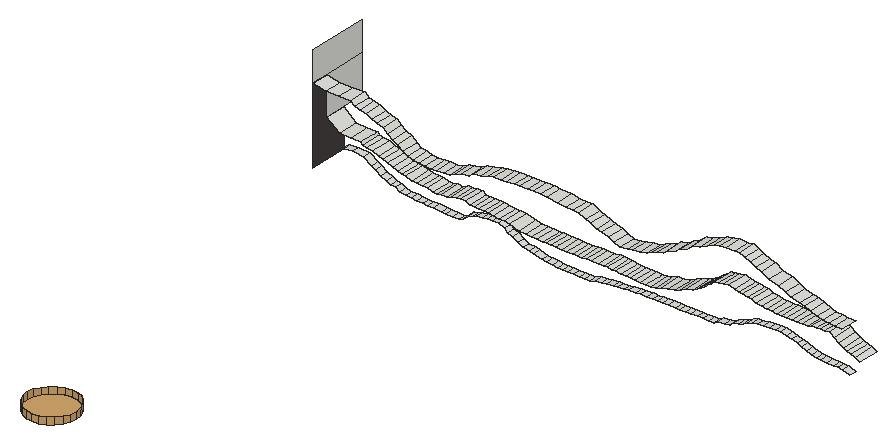
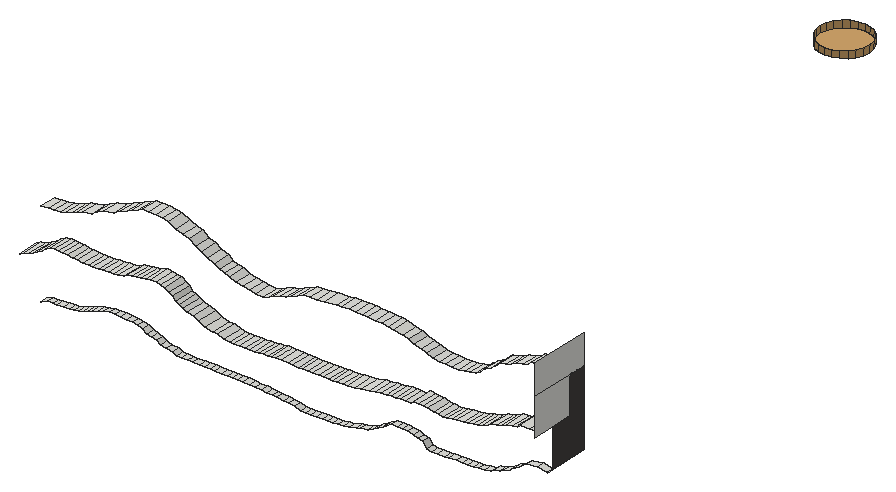
# SketchUp Ruby script. Lengths in inches.
U = 1.inch
M = Sketchup.active_model
def pt(a) = Geom::Point3d.new(a.map { |v| v * U })
def face(e, loops, mat)
  f = e.add_face(loops[0].map { |a| pt(a) })
  loops[1..].each { |l| e.add_face(l.map { |a| pt(a) }).erase! }
  f.material = f.back_material = mat if mat
  f
end
# faces: each face lists its corners as indices into pts; further lists are holes
def faces(e, pts, list, mat = nil) = list.each { |f| face(e, (f[0].is_a?(Array) ? f : [f]).map { |l| l.map { |i| pts[i] } }, mat) }
# xy, xz, yz: faces in a plane at the given z, y or x. An outline is a flat list of corners, or four numbers for a rectangle; further outlines are holes
def ring(l) = l.size == 4 ? [[l[0], l[1]], [l[2], l[1]], [l[2], l[3]], [l[0], l[3]]] : l.each_slice(2).to_a
def flat(e, list, mat, &to3) = list.each { |f| face(e, (f[0].is_a?(Array) ? f : [f]).map { |l| ring(l).map { |u, v| to3.(u, v) } }, mat) }
def xy(e, z, list, mat = nil) = flat(e, list, mat) { |x, y| [x, y, z] }
def xz(e, y, list, mat = nil) = flat(e, list, mat) { |x, z| [x, y, z] }
def yz(e, x, list, mat = nil) = flat(e, list, mat) { |y, z| [x, y, z] }
def lines(e, pts, list) = list.each { |a, b| e.add_line(pt(pts[a]), pt(pts[b])) }
# prism: a flat outline (further loops are holes) pulled along v
def prism(e, loops, v, mat = nil)
  f = face(e, loops, mat); d = Geom::Vector3d.new(v.map { |x| x * U })
  f.pushpull(f.normal.samedirection?(d) ? d.length : -d.length)
end
def box(e, o, s, mat = nil) = prism(e, [[o, [o[0] + s[0], o[1], o[2]], [o[0] + s[0], o[1] + s[1], o[2]], [o[0], o[1] + s[1], o[2]]]], [0, 0, s[2]], mat)
def at(x, y, z, deg = 0) = Geom::Transformation.translation(pt([x, y, z])) * Geom::Transformation.rotation(ORIGIN, Z_AXIS, deg.degrees)
def axes(o, x, y, z) = Geom::Transformation.new([*x, 0, *y, 0, *z, 0, *pt(o).to_a, 1])
def part(name) = M.definitions.add(name)
# library, detail: a bought-in or finely detailed component or shape, given as its bounding box
def library(name, o, s) = part(name).tap { |d| box(d.entities, o, s) }
def detail(e, o, s) = box(e.add_group.entities, o, s)
def put(e, d, t, mat = nil) = e.add_instance(d, t).tap { |i| i.material = mat if mat }
def group(e, t, mat = nil) = e.add_group.tap { |g| g.transformation = t; g.material = mat if mat }.entities
root = M.entities
M.materials.add("[Field Square Tile]").color = [211, 167, 108]
M.materials.add("[Granite Tile]1").color = [68, 65, 63]
xy(root,237.65,[[2039.58,2401.37,2040.27,2402.3],[2040.27,2401.37,2040.89,2402.3]])
xy(root,238.33,[[2048.68,2401.37,2049.23,2402.3],[2049.23,2401.37,2049.91,2402.3]])
xy(root,238.34,[[2050.59,2401.37,2051.52,2402.3],[2051.52,2401.37,2052.01,2402.3],[2052.01,2401.37,2052.77,2402.3],[2052.77,2401.37,2053.4,2402.3],[2053.4,2401.37,2054.15,2402.3],
  [2054.15,2401.37,2054.77,2402.3],[2054.77,2401.37,2055.54,2402.3],[2055.54,2401.37,2056.16,2402.3]])
xy(root,241.52,[[2010.28,2396.68,2010.34,2402.3]])
xy(root,241.68,[[2040.78,2398.8,2041.37,2401.37]])
xy(root,241.75,[[2043.13,2398.8,2044,2401.37],[2044,2398.8,2044.62,2401.37],[2044.62,2398.8,2045.13,2401.37]])
xy(root,250.6875,[[2030.6,2327.89,2029.81,2328,2029.07,2328.3,2028.43,2328.79,2027.95,2329.43,2027.64,2330.16,2027.54,2330.96,2027.64,2331.75,2027.95,2332.49,2028.43,2333.12,2029.07,2333.61,2029.81,2333.91,2030.6,2334.02,2031.39,2333.91,2032.13,2333.61,2032.76,2333.12,2033.25,2332.49,2033.56,2331.75,2033.66,2330.96,2033.56,2330.16,2033.25,2329.43,2032.76,2328.79,2032.13,2328.3,2031.39,2328]],"[Field Square Tile]")
xz(root,2396.68,[[2010.28,241.52,2010.34,251.5]])
yz(root,2010.34,[[2398.8,246.2,2404.3,250.88],[2396.68,250.88,2404.3,254.5]])
yz(root,2010.34,[[2396.68,241.52,2401.37,241.52,2401.37,246.2,2398.8,246.2,2398.8,250.88,2396.68,250.88]],"[Granite Tile]1")
p = [[2040.89,2401.37,237.65],[2040.89,2402.3,237.65],[2041.56,2402.3,237.89],[2041.56,2401.37,237.89],[2036.22,2401.37,237.76],[2036.22,2402.3,237.76],
  [2036.93,2402.3,237.71],[2036.93,2401.37,237.71],[2037.54,2402.3,237.68],[2037.54,2401.37,237.68],[2038.14,2402.3,237.67],[2038.14,2401.37,237.67],
  [2038.89,2402.3,237.66],[2038.89,2401.37,237.66],[2039.58,2402.3,237.65],[2039.58,2401.37,237.65],[2034.87,2401.37,237.9],[2034.87,2402.3,237.9],
  [2035.53,2402.3,237.82],[2035.53,2401.37,237.82],[2033.93,2401.37,238.21],[2033.93,2402.3,238.21],[2042.32,2402.3,237.94],[2042.32,2401.37,237.94],
  [2042.9375,2402.3,237.98],[2042.9375,2401.37,237.98],[2043.79,2402.3,238.1],[2043.79,2401.37,238.1],[2044.34,2402.3,238.13],[2044.34,2401.37,238.13],
  [2045.1,2402.3,238.15],[2045.1,2401.37,238.15],[2033.46,2401.37,238.31],[2033.46,2402.3,238.31],[2045.73,2402.3,238.26],[2045.73,2401.37,238.26],
  [2032.55,2401.37,238.43],[2032.55,2402.3,238.43],[2046.48,2402.3,238.28],[2046.48,2401.37,238.28],[2047.11,2402.3,238.3],[2047.11,2401.37,238.3],
  [2047.96,2402.3,238.32],[2047.96,2401.37,238.32],[2048.68,2402.3,238.33],[2048.68,2401.37,238.33],[2049.91,2401.37,238.33],[2049.91,2402.3,238.33],
  [2050.59,2402.3,238.34],[2050.59,2401.37,238.34],[2056.16,2401.37,238.34],[2056.16,2402.3,238.34],[2056.67,2402.3,238.59],[2056.67,2401.37,238.59],
  [2031.9,2401.37,238.74],[2031.9,2402.3,238.74],[2072.19,2401.37,238.78],[2072.19,2402.3,238.78],[2072.97,2402.3,238.43],[2072.97,2401.37,238.43],
  [2057.49,2402.3,238.72],[2057.49,2401.37,238.72],[2031.32,2401.37,239.11],[2031.32,2402.3,239.11],[2058.18,2402.3,238.86],[2058.18,2401.37,238.86],
  [2021.53,2401.37,238.92],[2021.53,2402.3,238.92],[2022.57,2402.3,238.82],[2022.57,2401.37,238.82],[2023.08,2402.3,238.8],[2023.08,2401.37,238.8],
  [2023.95,2402.3,238.79],[2023.95,2401.37,238.79],[2024.69,2402.3,238.77],[2024.69,2401.37,238.77],[2025.22,2402.3,238.9375],[2025.22,2401.37,238.9375],
  [2069.47,2401.37,238.875],[2069.47,2402.3,238.875],[2070.22,2402.3,238.83],[2070.22,2401.37,238.83],[2070.98,2402.3,238.8],[2070.98,2401.37,238.8],
  [2071.52,2402.3,238.79],[2071.52,2401.37,238.79],[2019.44,2401.37,238.97],[2019.44,2402.3,238.97],[2020.14,2402.3,238.94],[2020.14,2401.37,238.94],
  [2020.84,2402.3,238.93],[2020.84,2401.37,238.93],[2025.78,2402.3,239.55],[2025.78,2401.37,239.55],[2058.69,2402.3,239.18],[2058.69,2401.37,239.18],
  [2068.32,2401.37,239.04],[2068.32,2402.3,239.04],[2068.9,2402.3,238.94],[2068.9,2401.37,238.94],[2018.07,2401.37,239.09],[2018.07,2402.3,239.09],
  [2018.76,2402.3,239.03],[2018.76,2401.37,239.03],[2067.66,2401.37,239.29],[2067.66,2402.3,239.29],[2017.29,2401.37,239.19],[2017.29,2402.3,239.19],
  [2030.74,2401.37,239.38],[2030.74,2402.3,239.38],[2016.78,2401.37,239.52],[2016.78,2402.3,239.52],[2059.28,2402.3,239.35],[2059.28,2401.37,239.35],
  [2067.08,2401.37,239.53],[2067.08,2402.3,239.53],[2030.28,2401.37,239.71],[2030.28,2402.3,239.71],[2059.84,2402.3,239.52],[2059.84,2401.37,239.52],
  [2016.22,2401.37,239.64],[2016.22,2402.3,239.64],[2060.39,2402.3,239.85],[2060.39,2401.37,239.85],[2066.55,2401.37,239.7],[2066.55,2402.3,239.7],
  [2015.77,2401.37,239.86],[2015.77,2402.3,239.86],[2026.36,2402.3,239.69],[2026.36,2401.37,239.69],[2026.91,2402.3,239.88],[2026.91,2401.37,239.88],
  [2029.58,2401.37,240.11],[2029.58,2402.3,240.11],[2065.86,2401.37,239.92],[2065.86,2402.3,239.92],[2061.03,2402.3,240.03],[2061.03,2401.37,240.03],
  [2014.98,2401.37,240.2],[2014.98,2402.3,240.2],[2027.64,2402.3,239.99],[2027.64,2401.37,239.99],[2065.23,2401.37,240.11],[2065.23,2402.3,240.11],
  [2028.23,2402.3,240.05],[2028.23,2401.37,240.05],[2028.89,2402.3,240.09],[2028.89,2401.37,240.09],[2061.6875,2402.3,240.12],[2061.6875,2401.37,240.12],
  [2062.36,2402.3,240.19],[2062.36,2401.37,240.19],[2064.45,2401.37,240.27],[2064.45,2402.3,240.27],[2014.38,2401.37,240.59],[2014.38,2402.3,240.59],
  [2063.125,2402.3,240.23],[2063.125,2401.37,240.23],[2063.83,2402.3,240.25],[2063.83,2401.37,240.25],[2013.84,2401.37,240.85],[2013.84,2402.3,240.85],
  [2012.82,2401.37,241.55],[2012.82,2402.3,241.55],[2046.76,2398.8,241.57],[2046.76,2401.37,241.57],[2047.3,2401.37,241.53],[2047.3,2398.8,241.53],
  [2047.92,2401.37,241.51],[2047.92,2398.8,241.51],[2048.47,2401.37,241.49],[2048.47,2398.8,241.49],[2049.17,2401.37,241.48],[2049.17,2398.8,241.48],
  [2049.83,2401.37,241.47],[2049.83,2398.8,241.47],[2050.4,2401.37,241.46],[2050.4,2398.8,241.46],[2051.11,2401.37,241.6],[2051.11,2398.8,241.6],
  [2010.34,2401.37,241.52],[2010.34,2402.3,241.52],[2011.55,2402.3,241.69],[2011.55,2401.37,241.69],[2046.15,2398.8,241.66],[2046.15,2401.37,241.66],
  [2051.84,2401.37,241.85],[2051.84,2398.8,241.85],[2037.12,2398.8,241.75],[2037.12,2401.37,241.75],[2037.57,2401.37,241.74],[2037.57,2398.8,241.74],
  [2038.12,2401.37,241.72],[2038.12,2398.8,241.72],[2038.75,2401.37,241.71],[2038.75,2398.8,241.71],[2039.38,2401.37,241.7],[2039.38,2398.8,241.7],
  [2040.11,2401.37,241.69],[2040.11,2398.8,241.69],[2040.78,2401.37,241.68],[2040.78,2398.8,241.68],[2041.37,2398.8,241.68],[2041.37,2401.37,241.68],
  [2041.86,2401.37,241.67],[2041.86,2398.8,241.67],[2042.5625,2401.37,241.74],[2042.5625,2398.8,241.74],[2043.13,2401.37,241.75],[2043.13,2398.8,241.75],
  [2045.13,2398.8,241.75],[2045.13,2401.37,241.75],[2045.62,2401.37,241.67],[2045.62,2398.8,241.67],[2034.93,2398.8,241.89],[2034.93,2401.37,241.89],
  [2035.75,2401.37,241.83],[2035.75,2398.8,241.83],[2036.35,2401.37,241.78],[2036.35,2398.8,241.78],[2052.51,2401.37,241.91],[2052.51,2398.8,241.91],
  [2034.16,2398.8,241.96],[2034.16,2401.37,241.96],[2053.41,2401.37,242.1],[2053.41,2398.8,242.1],[2032.99,2398.8,242.24],[2032.99,2401.37,242.24],
  [2054.18,2401.37,242.46],[2054.18,2398.8,242.46],[2032.32,2398.8,242.34],[2032.32,2401.37,242.34],[2075.79,2398.8,242.51],[2075.79,2401.37,242.51],
  [2076.3,2401.37,242.21],[2076.3,2398.8,242.21],[2031.66,2398.8,242.38],[2031.66,2401.37,242.38],[2031,2398.8,242.48],[2031,2401.37,242.48],
  [2022.82,2398.8,242.68],[2022.82,2401.37,242.68],[2023.49,2401.37,242.51],[2023.49,2398.8,242.51],[2024.01,2401.37,242.46],[2024.01,2398.8,242.46],
  [2024.55,2401.37,242.58],[2024.55,2398.8,242.58],[2030.36,2398.8,242.57],[2030.36,2401.37,242.57],[2054.88,2401.37,242.78],[2054.88,2398.8,242.78],
  [2075.2,2398.8,242.68],[2075.2,2401.37,242.68],[2025.18,2401.37,242.57],[2025.18,2398.8,242.57],[2025.81,2401.37,242.81],[2025.81,2398.8,242.81],
  [2027.58,2398.8,242.92],[2027.58,2401.37,242.92],[2028.01,2401.37,242.625],[2028.01,2398.8,242.625],[2028.62,2401.37,242.65],[2028.62,2398.8,242.65],
  [2029.17,2401.37,242.62],[2029.17,2398.8,242.62],[2029.8,2401.37,242.58],[2029.8,2398.8,242.58],[2021.47,2398.8,242.78],[2021.47,2401.37,242.78],
  [2022.28,2401.37,242.73],[2022.28,2398.8,242.73],[2074.7,2398.8,242.875],[2074.7,2401.37,242.875],[2020.17,2398.8,243.06],[2020.17,2401.37,243.06],
  [2020.89,2401.37,242.85],[2020.89,2398.8,242.85],[2026.38,2401.37,242.86],[2026.38,2398.8,242.86],[2055.65,2401.37,242.97],[2055.65,2398.8,242.97],
  [2026.94,2401.37,242.89],[2026.94,2398.8,242.89],[2074.31,2398.8,243.09],[2074.31,2401.37,243.09],[2056.18,2401.37,243.23],[2056.18,2398.8,243.23],
  [2019.1,2398.8,243.3],[2019.1,2401.37,243.3],[2019.6875,2401.37,243.14],[2019.6875,2398.8,243.14],[2073.7,2398.8,243.43],[2073.7,2401.37,243.43],
  [2056.58,2401.37,243.48],[2056.58,2398.8,243.48],[2018.46,2398.8,243.48],[2018.46,2401.37,243.48],[2073.16,2398.8,243.8],[2073.16,2401.37,243.8],
  [2017.94,2398.8,243.79],[2017.94,2401.37,243.79],[2057.1,2401.37,243.72],[2057.1,2398.8,243.72],[2057.4375,2401.37,244.12],[2057.4375,2398.8,244.12],
  [2017.28,2398.8,243.95],[2017.28,2401.37,243.95],[2072.56,2398.8,244.18],[2072.56,2401.37,244.18],[2016.76,2398.8,244.11],[2016.76,2401.37,244.11],
  [2065.38,2398.8,243.99],[2065.38,2401.37,243.99],[2066.1,2401.37,243.95],[2066.1,2398.8,243.95],[2066.6,2401.37,243.93],[2066.6,2398.8,243.93],
  [2067.29,2401.37,243.91],[2067.29,2398.8,243.91],[2067.86,2401.37,243.89],[2067.86,2398.8,243.89],[2068.56,2401.37,243.88],[2068.56,2398.8,243.88],
  [2069.21,2401.37,243.94],[2069.21,2398.8,243.94],[2069.85,2401.37,243.95],[2069.85,2398.8,243.95],[2070.41,2401.37,244.1],[2070.41,2398.8,244.1],
  [2064.2,2398.8,244.11],[2064.2,2401.37,244.11],[2064.76,2401.37,244.04],[2064.76,2398.8,244.04],[2016.09,2398.8,244.41],[2016.09,2401.37,244.41],
  [2057.91,2401.37,244.39],[2057.91,2398.8,244.39],[2063.45,2398.8,244.25],[2063.45,2401.37,244.25],[2071.04,2401.37,244.13],[2071.04,2398.8,244.13],
  [2071.52,2401.37,244.15],[2071.52,2398.8,244.15],[2072.04,2401.37,244.17],[2072.04,2398.8,244.17],[2062.99,2398.8,244.51],[2062.99,2401.37,244.51],
  [2015.33,2398.8,244.54],[2015.33,2401.37,244.54],[2058.39,2401.37,244.73],[2058.39,2398.8,244.73],[2014.77,2398.8,244.61],[2014.77,2401.37,244.61],
  [2061.84,2398.8,244.67],[2061.84,2401.37,244.67],[2062.45,2401.37,244.55],[2062.45,2398.8,244.55],[2014.55,2398.8,244.92],[2014.55,2401.37,244.92],
  [2058.875,2401.37,244.87],[2058.875,2398.8,244.87],[2060.79,2398.8,244.81],[2060.79,2401.37,244.81],[2061.36,2401.37,244.7],[2061.36,2398.8,244.7],
  [2060.14,2398.8,245.01],[2060.14,2401.37,245.01],[2011.91,2398.8,244.96],[2011.91,2401.37,244.96],[2013.3,2401.37,244.9375],[2013.3,2398.8,244.9375],
  [2059.46,2401.37,244.95],[2059.46,2398.8,244.95],[2010.34,2398.8,246.2],[2010.34,2401.37,246.2],[2047.59,2396.68,246.35],[2047.59,2398.8,246.35],
  [2048.36,2398.8,246.05],[2048.36,2396.68,246.05],[2049.26,2398.8,246.13],[2049.26,2396.68,246.13],[2049.97,2398.8,246.29],[2049.97,2396.68,246.29],
  [2050.77,2398.8,246.41],[2050.77,2396.68,246.41],[2046.98,2396.68,246.66],[2046.98,2398.8,246.66],[2051.68,2398.8,246.55],[2051.68,2396.68,246.55],
  [2023.4,2396.68,246.62],[2023.4,2398.8,246.62],[2024.14,2398.8,246.54],[2024.14,2396.68,246.54],[2024.92,2398.8,246.51],[2024.92,2396.68,246.51],
  [2025.7,2398.8,246.58],[2025.7,2396.68,246.58],[2074.89,2396.68,246.59],[2074.89,2398.8,246.59],[2075.78,2398.8,246.55],[2075.78,2396.68,246.55],
  [2022.74,2396.68,246.73],[2022.74,2398.8,246.73],[2026.5,2398.8,246.59],[2026.5,2396.68,246.59],[2027.3,2398.8,246.69],[2027.3,2396.68,246.69],
  [2052.41,2398.8,246.92],[2052.41,2396.68,246.92],[2074.18,2396.68,246.66],[2074.18,2398.8,246.66],[2022.02,2396.68,246.88],[2022.02,2398.8,246.88],
  [2028.01,2398.8,247.03],[2028.01,2396.68,247.03],[2046.125,2396.68,246.94],[2046.125,2398.8,246.94],[2073.39,2396.68,246.75],[2073.39,2398.8,246.75],
  [2072.7,2396.68,246.95],[2072.7,2398.8,246.95],[2021.47,2396.68,247.25],[2021.47,2398.8,247.25],[2045.44,2396.68,247.08],[2045.44,2398.8,247.08],
  [2053.02,2398.8,247.12],[2053.02,2396.68,247.12],[2028.7,2398.8,247.2],[2028.7,2396.68,247.2],[2071.89,2396.68,247.25],[2071.89,2398.8,247.25],
  [2044.76,2396.68,247.46],[2044.76,2398.8,247.46],[2053.7,2398.8,247.31],[2053.7,2396.68,247.31],[2029.67,2398.8,247.39],[2029.67,2396.68,247.39],
  [2071.21,2396.68,247.53],[2071.21,2398.8,247.53],[2020.83,2396.68,247.72],[2020.83,2398.8,247.72],[2054.27,2398.8,247.71],[2054.27,2396.68,247.71],
  [2030.3,2398.8,247.78],[2030.3,2396.68,247.78],[2044.13,2396.68,247.66],[2044.13,2398.8,247.66],[2070.63,2396.68,247.66],[2070.63,2398.8,247.66],
  [2020.18,2396.68,248.07],[2020.18,2398.8,248.07],[2043.29,2396.68,248.08],[2043.29,2398.8,248.08],[2055.2,2398.8,248.03],[2055.2,2396.68,248.03],
  [2069.5,2396.68,247.9],[2069.5,2398.8,247.9],[2031.08,2398.8,247.89],[2031.08,2396.68,247.89],[2032.08,2398.8,248.18],[2032.08,2396.68,248.18],
  [2068.9,2396.68,248.26],[2068.9,2398.8,248.26],[2055.91,2398.8,248.46],[2055.91,2396.68,248.46],[2019.55,2396.68,248.51],[2019.55,2398.8,248.51],
  [2041.67,2396.68,248.15],[2041.67,2398.8,248.15],[2042.49,2398.8,248.11],[2042.49,2396.68,248.11],[2032.72,2398.8,248.29],[2032.72,2396.68,248.29],
  [2040.64,2396.68,248.28],[2040.64,2398.8,248.28],[2033.61,2398.8,248.35],[2033.61,2396.68,248.35],[2039.24,2396.68,248.39],[2039.24,2398.8,248.39],
  [2067.99,2396.68,248.69],[2067.99,2398.8,248.69],[2034.34,2398.8,248.4],[2034.34,2396.68,248.4],[2035.33,2398.8,248.4375],[2035.33,2396.68,248.4375],
  [2035.99,2398.8,248.46],[2035.99,2396.68,248.46],[2038.51,2396.68,248.49],[2038.51,2398.8,248.49],[2019.06,2396.68,249.01],[2019.06,2398.8,249.01],
  [2036.88,2398.8,248.47],[2036.88,2396.68,248.47],[2037.62,2398.8,248.48],[2037.62,2396.68,248.48],[2056.69,2398.8,248.82],[2056.69,2396.68,248.82],
  [2066.77,2396.68,248.95],[2066.77,2398.8,248.95],[2057.41,2398.8,249.37],[2057.41,2396.68,249.37],[2065.88,2396.68,249.46],[2065.88,2398.8,249.46],
  [2018.29,2396.68,249.2],[2018.29,2398.8,249.2],[2017.62,2396.68,249.41],[2017.62,2398.8,249.41],[2016.95,2396.68,249.8],[2016.95,2398.8,249.8],
  [2058.2,2398.8,249.5625],[2058.2,2396.68,249.5625],[2065.12,2396.68,249.68],[2065.12,2398.8,249.68],[2059.1,2398.8,249.9],[2059.1,2396.68,249.9],
  [2064.46,2396.68,250.0625],[2064.46,2398.8,250.0625],[2016.15,2396.68,249.97],[2016.15,2398.8,249.97],[2060.02,2398.8,250.35],[2060.02,2396.68,250.35],
  [2015.54,2396.68,250.15],[2015.54,2398.8,250.15],[2015.01,2396.68,250.55],[2015.01,2398.8,250.55],[2063.77,2396.68,250.32],[2063.77,2398.8,250.32],
  [2060.68,2398.8,250.49],[2060.68,2396.68,250.49],[2063.15,2396.68,250.61],[2063.15,2398.8,250.61],[2010.34,2396.68,250.88],[2010.34,2398.8,250.88],
  [2011.93,2398.8,250.53],[2011.93,2396.68,250.53],[2013.55,2398.8,250.54],[2013.55,2396.68,250.54],[2061.49,2398.8,250.6],[2061.49,2396.68,250.6],
  [2062.51,2398.8,250.58],[2062.51,2396.68,250.58],[2030.6,2327.89,251.5],[2029.81,2328,251.5],[2029.81,2328,250.6875],[2030.6,2327.89,250.6875],
  [2031.39,2328,251.5],[2031.39,2328,250.6875],[2029.07,2328.3,251.5],[2029.07,2328.3,250.6875],[2032.13,2328.3,251.5],[2032.13,2328.3,250.6875],
  [2028.43,2328.79,251.5],[2028.43,2328.79,250.6875],[2032.76,2328.79,251.5],[2032.76,2328.79,250.6875],[2027.95,2329.43,251.5],[2027.95,2329.43,250.6875],
  [2033.25,2329.43,251.5],[2033.25,2329.43,250.6875],[2027.64,2330.16,251.5],[2027.64,2330.16,250.6875],[2033.56,2330.16,251.5],[2033.56,2330.16,250.6875],
  [2027.54,2330.96,251.5],[2027.54,2330.96,250.6875],[2033.66,2330.96,251.5],[2033.66,2330.96,250.6875],[2027.64,2331.75,251.5],[2027.64,2331.75,250.6875],
  [2033.56,2331.75,251.5],[2033.56,2331.75,250.6875],[2027.95,2332.49,251.5],[2027.95,2332.49,250.6875],[2033.25,2332.49,251.5],[2033.25,2332.49,250.6875],
  [2028.43,2333.12,251.5],[2028.43,2333.12,250.6875],[2032.76,2333.12,251.5],[2032.76,2333.12,250.6875],[2029.07,2333.61,251.5],[2029.07,2333.61,250.6875],
  [2032.13,2333.61,251.5],[2032.13,2333.61,250.6875],[2029.81,2333.91,251.5],[2029.81,2333.91,250.6875],[2031.39,2333.91,251.5],[2031.39,2333.91,250.6875],
  [2030.6,2334.02,251.5],[2030.6,2334.02,250.6875]]
faces(root,p,[[0,1,2,3],[4,5,6,7],[7,6,8,9],[9,8,10,11],[11,10,12,13],[13,12,14,15],[16,17,18,19],[19,18,5,4],
  [20,21,17,16],[3,2,22,23],[23,22,24,25],[25,24,26,27],[27,26,28,29],[29,28,30,31],[32,33,21,20],[31,30,34,35],
  [36,37,33,32],[35,34,38,39],[39,38,40,41],[41,40,42,43],[43,42,44,45],[46,47,48,49],[50,51,52,53],[54,55,37,36],
  [56,57,58,59],[53,52,60,61],[62,63,55,54],[61,60,64,65],[66,67,68,69],[69,68,70,71],[71,70,72,73],[73,72,74,75],
  [75,74,76,77],[78,79,80,81],[81,80,82,83],[83,82,84,85],[85,84,57,56],[86,87,88,89],[89,88,90,91],[91,90,67,66],
  [77,76,92,93],[65,64,94,95],[96,97,98,99],[99,98,79,78],[100,101,102,103],[103,102,87,86],[104,105,97,96],[106,107,101,100],
  [108,109,63,62],[110,111,107,106],[95,94,112,113],[114,115,105,104],[116,117,109,108],[113,112,118,119],[120,121,111,110],[119,118,122,123],
  [124,125,115,114],[126,127,121,120],[93,92,128,129],[129,128,130,131],[132,133,117,116],[134,135,125,124],[123,122,136,137],[138,139,127,126],
  [131,130,140,141],[142,143,135,134],[141,140,144,145],[145,144,146,147],[137,136,148,149],[147,146,133,132],[149,148,150,151],[152,153,143,142],
  [154,155,139,138],[151,150,156,157],[157,156,158,159],[159,158,153,152],[160,161,155,154],[162,163,161,160],[164,165,166,167],[167,166,168,169],
  [169,168,170,171],[171,170,172,173],[173,172,174,175],[175,174,176,177],[177,176,178,179],[180,181,182,183],[184,185,165,164],[179,178,186,187],
  [183,182,163,162],[188,189,190,191],[191,190,192,193],[193,192,194,195],[195,194,196,197],[197,196,198,199],[199,198,200,201],[202,203,204,205],
  [205,204,206,207],[207,206,208,209],[210,211,212,213],[213,212,185,184],[214,215,216,217],[217,216,218,219],[219,218,189,188],[187,186,220,221],
  [222,223,215,214],[221,220,224,225],[226,227,223,222],[225,224,228,229],[230,231,227,226],[232,233,234,235],[236,237,231,230],[238,239,237,236],
  [240,241,242,243],[243,242,244,245],[245,244,246,247],[248,249,239,238],[229,228,250,251],[252,253,233,232],[247,246,254,255],[255,254,256,257],
  [258,259,260,261],[261,260,262,263],[263,262,264,265],[265,264,266,267],[267,266,249,248],[268,269,270,271],[271,270,241,240],[272,273,253,252],
  [274,275,276,277],[277,276,269,268],[257,256,278,279],[251,250,280,281],[279,278,282,283],[283,282,259,258],[284,285,273,272],[281,280,286,287],
  [288,289,290,291],[291,290,275,274],[292,293,285,284],[287,286,294,295],[296,297,289,288],[298,299,293,292],[300,301,297,296],[295,294,302,303],
  [303,302,304,305],[306,307,301,300],[308,309,299,298],[310,311,307,306],[312,313,314,315],[315,314,316,317],[317,316,318,319],[319,318,320,321],
  [321,320,322,323],[323,322,324,325],[325,324,326,327],[327,326,328,329],[330,331,332,333],[333,332,313,312],[334,335,311,310],[305,304,336,337],
  [338,339,331,330],[329,328,340,341],[341,340,342,343],[343,342,344,345],[345,344,309,308],[346,347,339,338],[348,349,335,334],[337,336,350,351],
  [352,353,349,348],[354,355,356,357],[357,356,347,346],[358,359,353,352],[351,350,360,361],[362,363,364,365],[365,364,355,354],[366,367,363,362],
  [368,369,370,371],[371,370,359,358],[361,360,372,373],[373,372,367,366],[374,375,369,368],[376,377,378,379],[379,378,380,381],[381,380,382,383],
  [383,382,384,385],[386,387,377,376],[385,384,388,389],[390,391,392,393],[393,392,394,395],[395,394,396,397],[398,399,400,401],[402,403,391,390],
  [397,396,404,405],[405,404,406,407],[389,388,408,409],[410,411,399,398],[412,413,403,402],[407,406,414,415],[416,417,387,386],[418,419,411,410],
  [420,421,419,418],[422,423,413,412],[424,425,417,416],[409,408,426,427],[415,414,428,429],[430,431,421,420],[432,433,425,424],[427,426,434,435],
  [429,428,436,437],[438,439,431,430],[440,441,423,422],[435,434,442,443],[437,436,444,445],[446,447,433,432],[448,449,439,438],[450,451,441,440],
  [452,453,447,446],[443,442,454,455],[456,457,449,448],[445,444,458,459],[459,458,460,461],[462,463,457,456],[455,454,464,465],[466,467,451,450],
  [468,469,470,471],[471,470,453,452],[461,460,472,473],[474,475,469,468],[473,472,476,477],[478,479,475,474],[480,481,463,462],[477,476,482,483],
  [483,482,484,485],[485,484,486,487],[488,489,479,478],[490,491,467,466],[487,486,492,493],[493,492,494,495],[495,494,489,488],[465,464,496,497],
  [498,499,481,480],[497,496,500,501],[502,503,499,498],[504,505,491,490],[506,507,505,504],[508,509,507,506],[501,500,510,511],[512,513,503,502],
  [511,510,514,515],[516,517,513,512],[518,519,509,508],[515,514,520,521],[522,523,519,518],[524,525,523,522],[526,527,517,516],[521,520,528,529],
  [530,531,527,526],[532,533,534,535],[535,534,536,537],[537,536,525,524],[529,528,538,539],[539,538,540,541],[541,540,531,530]])
faces(root,p,[[542,543,544,545],[546,542,545,547],[543,548,549,544],[550,546,547,551],[548,552,553,549],[554,550,551,555],[552,556,557,553],[558,554,555,559],
  [556,560,561,557],[562,558,559,563],[560,564,565,561],[566,562,563,567],[564,568,569,565],[570,566,567,571],[568,572,573,569],[574,570,571,575],
  [572,576,577,573],[578,574,575,579],[576,580,581,577],[582,578,579,583],[580,584,585,581],[586,582,583,587],[584,588,589,585],[588,586,587,589]],"[Field Square Tile]")
